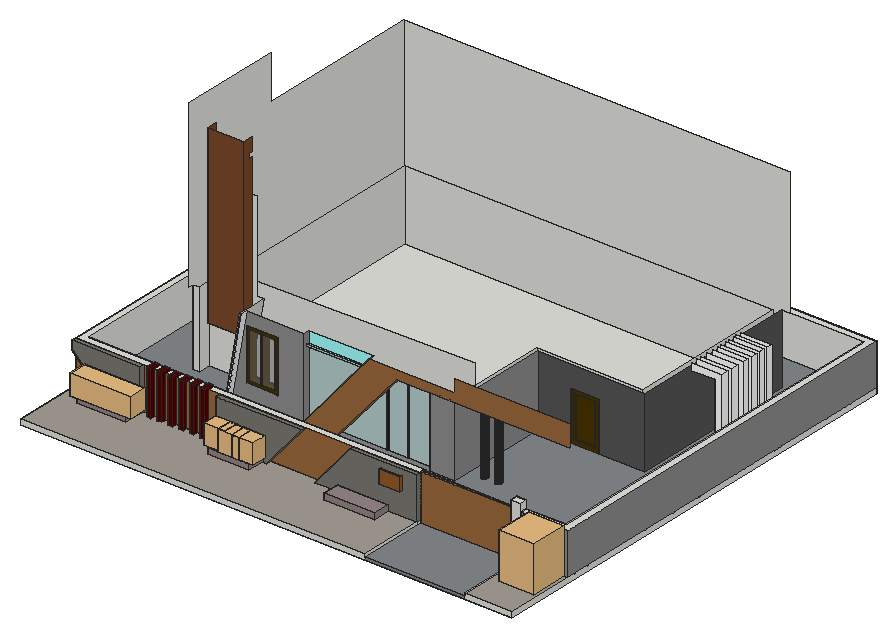
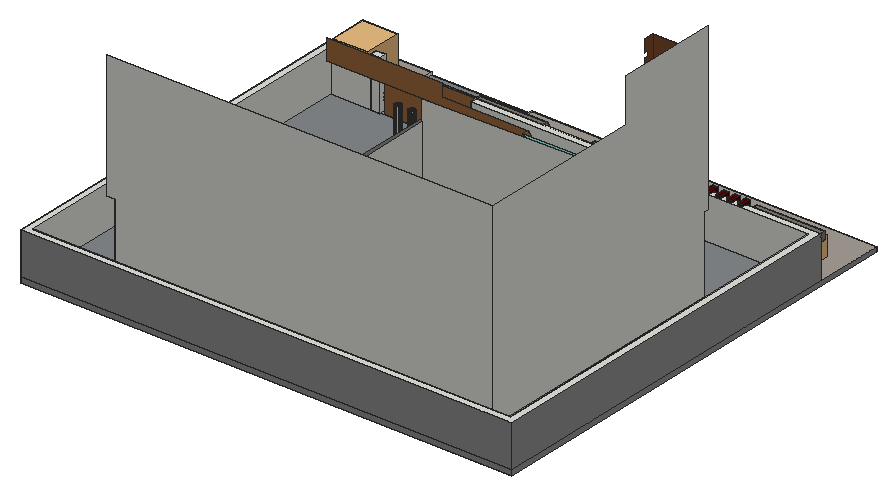
# SketchUp Ruby script. Lengths in inches.
U = 1.inch
M = Sketchup.active_model
def pt(a) = Geom::Point3d.new(a.map { |v| v * U })
def face(e, loops, mat)
  f = e.add_face(loops[0].map { |a| pt(a) })
  loops[1..].each { |l| e.add_face(l.map { |a| pt(a) }).erase! }
  f.material = f.back_material = mat if mat
  f
end
# faces: each face lists its corners as indices into pts; further lists are holes
def faces(e, pts, list, mat = nil) = list.each { |f| face(e, (f[0].is_a?(Array) ? f : [f]).map { |l| l.map { |i| pts[i] } }, mat) }
# xy, xz, yz: faces in a plane at the given z, y or x. An outline is a flat list of corners, or four numbers for a rectangle; further outlines are holes
def ring(l) = l.size == 4 ? [[l[0], l[1]], [l[2], l[1]], [l[2], l[3]], [l[0], l[3]]] : l.each_slice(2).to_a
def flat(e, list, mat, &to3) = list.each { |f| face(e, (f[0].is_a?(Array) ? f : [f]).map { |l| ring(l).map { |u, v| to3.(u, v) } }, mat) }
def xy(e, z, list, mat = nil) = flat(e, list, mat) { |x, y| [x, y, z] }
def xz(e, y, list, mat = nil) = flat(e, list, mat) { |x, z| [x, y, z] }
def yz(e, x, list, mat = nil) = flat(e, list, mat) { |y, z| [x, y, z] }
def lines(e, pts, list) = list.each { |a, b| e.add_line(pt(pts[a]), pt(pts[b])) }
# prism: a flat outline (further loops are holes) pulled along v
def prism(e, loops, v, mat = nil)
  f = face(e, loops, mat); d = Geom::Vector3d.new(v.map { |x| x * U })
  f.pushpull(f.normal.samedirection?(d) ? d.length : -d.length)
end
def box(e, o, s, mat = nil) = prism(e, [[o, [o[0] + s[0], o[1], o[2]], [o[0] + s[0], o[1] + s[1], o[2]], [o[0], o[1] + s[1], o[2]]]], [0, 0, s[2]], mat)
def at(x, y, z, deg = 0) = Geom::Transformation.translation(pt([x, y, z])) * Geom::Transformation.rotation(ORIGIN, Z_AXIS, deg.degrees)
def axes(o, x, y, z) = Geom::Transformation.new([*x, 0, *y, 0, *z, 0, *pt(o).to_a, 1])
def part(name) = M.definitions.add(name)
# library, detail: a bought-in or finely detailed component or shape, given as its bounding box
def library(name, o, s) = part(name).tap { |d| box(d.entities, o, s) }
def detail(e, o, s) = box(e.add_group.entities, o, s)
def put(e, d, t, mat = nil) = e.add_instance(d, t).tap { |i| i.material = mat if mat }
def group(e, t, mat = nil) = e.add_group.tap { |g| g.transformation = t; g.material = mat if mat }.entities
root = M.entities
M.materials.add("[Asphalt Stamped Brick]").color = [149, 133, 134]
M.materials.add("[Blacktop Old 01]").color = [132, 136, 139]
M.materials.add("[Carrera Marble]").color = [182, 207, 207]
M.materials.add("[Color A08]").color = [86, 0, 0]
M.materials.add("[Color C08]").color = [74, 51, 0]
M.materials.add("[Color H03]").color = [162, 255, 255]
M.materials.add("[Color M00]").color = [255, 255, 255]
M.materials.add("[Color M04]").color = [142, 142, 142]
M.materials.add("[Color M06]").color = [86, 86, 86]
M.materials.add("[Color M08]").color = [30, 30, 30]
M.materials.add("[Groundcover Sand Raked]").color = [165, 158, 150]
M.materials.add("[Rough Square Concrete Block]").color = [123, 120, 113]
M.materials.add("[Translucent Glass Gray]").color = [128, 128, 128]
M.materials["[Translucent Glass Gray]"].alpha = 0.5
M.materials.add("[Wood Floor Dark]").color = [123, 73, 42]
M.materials.add("[Wood Floor Parquet]").color = [145, 89, 39]
M.materials.add("[Wood Floor]").color = [155, 105, 61]
c1 = library("Plant\#1",[-5.68,0.72,0],[60.25,63.89,77.61])
c2 = library("FOLHAGEM DECORAÇÃO",[-6.77,-5.96,0],[13.85,12.76,12.48])
c3 = library("Group\#9",[0,0,0],[102.88,30.52,34.18])
xy(root,0,[[0,0,840,778.75]])
xy(root,4.5625,[[588.97,0,759.97,0,759.97,118.75,743.35,118.75,743.35,130.75,588.97,130.75]],"[Blacktop Old 01]")
xy(root,7.5625,[[126.8,110.75,134.92,116.58]],"[Color A08]")
xy(root,8.8125,[[163.67,110.75,171.8,116.58]],"[Color A08]")
xy(root,9,[[57.9,110.5625,115.8,118.75],[245.73,110.5625,333.45,118.75],[415,110.5625,564.34,118.75],[564.34,110.5625,588.97,118.75],[0,118.75,0,778.75,840,778.75,840,118.75,759.97,118.75,759.97,130.75,828,130.75,828,766.75,12,766.75,12,130.75,588.97,130.75,588.97,118.75],
  [743.35,118.75,759.97,130.75],[177.64,231,177.64,241.25,174.375,241.25,174.375,250.25,551.08,250.25,551.08,414.375,613.375,414.375,613.375,408.375,557.08,408.375,557.08,241.25,358.24,241.25,358.24,231],[514.48,231,557.08,241.25],[94.75,250.25,94.75,700.8125,741.0625,700.8125,741.0625,408.375,661.375,408.375,661.375,414.375,732.0625,414.375,732.0625,691.8125,103.75,691.8125,103.75,271.1875,105.9,271.1875,105.9,250.25],[174.375,250.25,551.08,250.25,551.08,281.3125,103.75,271.1875,174.375,271.1875],
  [582.5,258.46,581.04,258.72,579.69,259.34,578.55,260.29,577.7,261.51,577.18,262.9,577.05,264.38,577.3,265.84,577.93,267.1875,578.88,268.33,580.09,269.18,581.49,269.69,582.97,269.83,584.43,269.57,585.78,268.95,586.92,268,587.77,266.78,588.28,265.39,588.42,263.91,588.16,262.45,587.54,261.1,586.59,259.96,585.375,259.11,583.98,258.6],[605.875,258.46,604.41,258.72,603.07,259.34,601.93,260.29,601.07,261.51,600.56,262.9,600.43,264.38,600.68,265.84,601.3,267.1875,602.25,268.33,603.47,269.18,604.86,269.69,606.34,269.83,607.8,269.57,609.15,268.95,610.29,268,611.15,266.78,611.66,265.39,611.79,263.91,611.54,262.45,610.91,261.1,609.96,259.96,608.75,259.11,607.35,258.6],[103.75,271.1875,551.08,281.3125,551.08,414.375,732.0625,414.375,732.0625,691.8125,103.75,691.8125]])
xy(root,9,[[31.99,81.6875,115.8,110.5625],[255.9,81.6875,325.28,110.5625],[453.41,81.6875,540.22,110.5625]],"[Asphalt Stamped Brick]")
xy(root,9,[[[12,130.75,828,766.75],[174.375,220.625,174.375,271.1875,105.9,271.1875,105.9,250.25,94.75,250.25,94.75,700.8125,741.0625,700.8125,741.0625,408.375,661.375,408.375,661.375,414.375,613.375,414.375,613.375,408.375,557.08,408.375,557.08,231,514.48,231,514.48,241.25,471.69,241.25,471.69,240.4375,469.85,240.4375,469.85,241.25,436.25,241.25,436.25,240.4375,434.61,240.4375,434.61,241.25,358.24,241.25,358.24,231,177.64,231,177.64,220.625],[793.62,490.78,806.8125,502.66],[793.62,511.53,806.8125,523.41],[793.62,536.43,806.8125,546.3],[793.62,554.3,806.8125,564.18],[793.62,570.62,806.8125,580.49],[793.62,586.05,806.8125,595.93],[582.5,258.46,581.04,258.72,579.69,259.34,578.55,260.29,577.7,261.51,577.18,262.9,577.05,264.38,577.3,265.84,577.93,267.1875,578.88,268.33,580.09,269.18,581.49,269.69,582.97,269.83,584.43,269.57,585.78,268.95,586.92,268,587.77,266.78,588.28,265.39,588.42,263.91,588.16,262.45,587.54,261.1,586.59,259.96,585.375,259.11,583.98,258.6],[605.875,258.46,604.41,258.72,603.07,259.34,601.93,260.29,601.07,261.51,600.56,262.9,600.43,264.38,600.68,265.84,601.3,267.1875,602.25,268.33,603.47,269.18,604.86,269.69,606.34,269.83,607.8,269.57,609.15,268.95,610.29,268,611.15,266.78,611.66,265.39,611.79,263.91,611.54,262.45,610.91,261.1,609.96,259.96,608.75,259.11,607.35,258.6]]],"[Blacktop Old 01]")
xy(root,9,[[174.375,220.625,177.64,241.25]],"[Color M00]")
xy(root,9,[[434.61,240.4375,436.25,241.25],[469.85,240.4375,471.69,241.25]],"[Color M08]")
xy(root,9,[[[0,0,588.97,0,588.97,110.5625,540.22,110.5625,540.22,81.6875,453.41,81.6875,453.41,110.5625,415,110.5625,415,118.75,333.45,118.75,333.45,110.5625,325.28,110.5625,325.28,81.6875,255.9,81.6875,255.9,110.5625,245.73,110.5625,245.73,118.75,115.8,118.75,115.8,81.6875,31.99,81.6875,31.99,110.5625,57.9,110.5625,57.9,118.75,0,118.75],[145.23,110.75,153.36,116.58],[182.11,110.75,190.23,116.58],[200.55,110.75,208.67,116.58],[218.98,110.75,227.11,116.58]],[759.97,0,840,118.75]],"[Groundcover Sand Raked]")
xy(root,18.8125,[[31.99,81.6875,115.8,110.5625],[255.9,81.6875,325.28,110.5625],[453.41,81.6875,540.22,110.5625]],"[Asphalt Stamped Brick]")
xy(root,33.04,[[201.66,231,254.6,250.25]])
xy(root,48.51,[[527.14,106,563.34,110.5625]],"[Wood Floor Parquet]")
xy(root,70.88,[[527.14,106,563.34,110.5625]],"[Wood Floor Parquet]")
xy(root,81,[[0,118.75,126.8,118.75,126.8,127.97,134.92,127.97,134.92,118.75,145.23,118.75,145.23,127.97,153.36,127.97,153.36,118.75,163.67,118.75,163.67,127.97,171.8,127.97,171.8,118.75,182.11,118.75,182.11,127.97,190.23,127.97,190.23,118.75,200.55,118.75,200.55,127.97,208.67,127.97,208.67,118.75,218.98,118.75,218.98,127.97,227.11,127.97,227.11,118.75,588.97,118.75,588.97,130.75,12,130.75,12,766.75,828,766.75,828,130.75,759.97,130.75,759.97,118.75,840,118.75,840,778.75,0,778.75]])
xy(root,81,[[126.8,116.58,134.92,118.75],[145.23,116.58,153.36,118.75],[163.67,116.58,171.8,118.75],[182.11,116.58,190.23,118.75],[200.55,116.58,208.67,118.75],
  [218.98,116.58,227.11,118.75],[163.67,118.75,171.8,127.97],[182.11,118.75,190.23,127.97],[200.55,118.75,208.67,127.97],[218.98,118.75,227.11,127.97]],"[Color A08]")
xy(root,81,[[0,110.5625,115.8,118.75],[245.73,110.5625,393.07,118.75],[474.17,110.5625,588.97,118.75]],"[Rough Square Concrete Block]")
xy(root,84.3125,[[126.8,110.75,134.92,127.97],[145.23,110.75,153.36,127.97],[163.67,110.75,171.8,127.97],[182.11,110.75,190.23,127.97],[200.55,110.75,208.67,127.97],
  [218.98,110.75,227.11,127.97]],"[Color A08]")
xy(root,85.375,[[116.625,255.4375,178.1875,271.1875]])
xy(root,93,[[613.375,408.375,661.375,414.375]])
xy(root,94.25,[[743.35,118.75,759.97,130.75]])
xy(root,121.98,[[201.66,231,254.6,250.25]])
xy(root,122.22,[[299.43,236.6875,393.28,241.25]],"[Carrera Marble]")
xy(root,124.82,[[299.43,236.6875,395.4375,241.25]],"[Carrera Marble]")
xz(root,0,[[0,0,588.97,9],[759.97,0,840,9]])
xz(root,0,[[588.97,0,759.97,4.5625]],"[Blacktop Old 01]")
xz(root,81.6875,[[31.99,9,115.8,18.8125],[255.9,9,325.28,18.8125],[453.41,9,540.22,18.8125]],"[Asphalt Stamped Brick]")
xz(root,106,[[527.14,48.51,563.34,70.88]],"[Wood Floor Parquet]")
xz(root,110.5625,[[31.99,9,31.99,18.8125,48.09,18.8125,57.9,9],[57.9,9,115.8,18.8125],[255.9,9,325.28,18.8125],[453.41,9,540.22,18.8125]],"[Asphalt Stamped Brick]")
xz(root,110.5625,[[57.9,9,57.9,18.8125,48.09,18.8125],[245.73,9,255.9,9,255.9,18.8125,325.28,18.8125,325.28,9,333.45,9,393.07,81,245.73,81],[[415,9,453.41,9,453.41,18.8125,540.22,18.8125,540.22,9,588.97,9,588.97,81,474.17,81],[527.14,48.51,563.34,70.88]],[48.09,18.8125,115.8,18.8125,115.8,81,0,81,0,66.9]],"[Rough Square Concrete Block]")
xz(root,110.5625,[[527.14,48.51,563.34,70.88]],"[Wood Floor Parquet]")
xz(root,110.75,[[126.8,7.5625,134.92,84.3125],[163.67,8.8125,171.8,84.3125],[145.23,9,153.36,84.3125],[182.11,9,190.23,84.3125],[200.55,9,208.67,84.3125],
  [218.98,9,227.11,84.3125]],"[Color A08]")
xz(root,116.58,[[126.8,7.5625,134.92,81],[163.67,8.8125,171.8,81],[145.23,9,153.36,81],[182.11,9,190.23,81],[200.55,9,208.67,81],
  [218.98,9,227.11,81]],"[Color A08]")
xz(root,118.75,[[743.35,4.5625,759.97,9],[57.9,9,0,66.9,0,81,115.8,81,115.8,9],[245.73,9,245.73,81,393.07,81,333.45,9],[415,9,474.17,81,588.97,81,588.97,9],[743.35,9,759.97,94.25]])
xz(root,118.75,[[759.97,9,840,81]],"[Color M04]")
xz(root,118.75,[[0,9,57.9,9,0,66.9],[115.8,9,245.73,81],[333.45,9,415,9,474.17,81,393.07,81]],"[Wood Floor]")
xz(root,127.97,[[126.8,81,134.92,84.3125],[145.23,81,153.36,84.3125],[163.67,81,171.8,84.3125],[182.11,81,190.23,84.3125],[200.55,81,208.67,84.3125],
  [218.98,81,227.11,84.3125]],"[Color A08]")
xz(root,130.75,[[588.97,4.5625,743.35,9],[12,9,588.97,81],[743.35,9,759.97,94.25],[759.97,9,828,81]])
xz(root,220.625,[[174.375,9,177.64,9,201.89,143.5625,198.68,143.5625]],"[Color M00]")
xz(root,231,[[[177.64,9,201.89,143.5625,299.43,143.5625,299.43,9],[201.66,33.04,254.6,121.98]],[514.48,9,557.08,129]],"[Color M04]")
xz(root,231,[[299.43,9,358.24,9,458.61,129,754.5,129,754.5,165,557.08,165,557.08,143.5625,410.97,143.5625]],"[Wood Floor]")
xz(root,236.6875,[[299.43,122.22,393.28,122.22,395.4375,124.82,299.43,124.82]],"[Carrera Marble]")
xz(root,240.4375,[[434.61,9,436.25,9,436.25,102.26,434.61,100.3],[469.85,9,471.69,129]],"[Color M08]")
xz(root,241.25,[[299.43,9,393.28,122.22,299.43,122.22],[358.24,9,434.61,9,434.61,100.3],[436.25,9,469.85,9,469.85,129,458.61,129,436.25,102.26],[471.69,9,514.48,129]],"[Carrera Marble]")
xz(root,241.25,[[299.43,124.82,395.4375,124.82,410.97,143.5625,299.43,143.5625]],"[Color H03]")
xz(root,241.25,[[434.61,9,434.61,100.3,436.25,102.26,436.25,9],[469.85,9,471.69,129]],"[Color M08]")
xz(root,250.25,[[94.75,9,105.9,138.0625]])
xz(root,255.4375,[[116.625,85.375,178.1875,383.8125]],"[Wood Floor Dark]")
xz(root,271.1875,[[103.75,9,105.9,129],[105.9,9,174.375,9,198.68,143.5625,186.49,143.5625,186.49,297,178.1875,297,178.1875,85.375,116.625,85.375,116.625,357,105.9,357]])
xz(root,408.375,[[557.08,9,613.375,9,613.375,93,661.375,93,661.375,9,741.0625,9,741.0625,129,557.08,129]],"[Color M06]")
xz(root,414.375,[[551.08,9,551.08,129,732.0625,129,732.0625,9,661.375,9,661.375,93,613.375,93,613.375,9]])
xz(root,490.78,[[793.62,9,806.8125,9,806.8125,144.7,754.5,144.7,754.5,132.83,793.62,132.83]],"[Color M00]")
xz(root,502.66,[[793.62,9,793.62,132.83,754.5,132.83,754.5,144.7,806.8125,144.7,806.8125,9]],"[Color M00]")
xz(root,511.53,[[793.62,9,806.8125,9,806.8125,144.7,754.5,144.7,754.5,132.83,793.62,132.83]],"[Color M00]")
xz(root,523.41,[[793.62,9,793.62,132.83,754.5,132.83,754.5,144.7,806.8125,144.7,806.8125,9]],"[Color M00]")
xz(root,536.43,[[793.62,9,806.8125,9,806.8125,144.7,754.5625,144.7,754.5625,133.42,793.62,133.42]],"[Color M00]")
xz(root,546.3,[[793.62,9,793.62,133.42,754.5625,133.42,754.5625,144.7,806.8125,144.7,806.8125,9]],"[Color M00]")
xz(root,554.3,[[793.62,9,806.8125,9,806.8125,144.7,754.5625,144.7,754.5625,133.42,793.62,133.42]],"[Color M00]")
xz(root,564.18,[[793.62,9,793.62,133.42,754.5625,133.42,754.5625,144.7,806.8125,144.7,806.8125,9]],"[Color M00]")
xz(root,570.62,[[793.62,9,806.8125,9,806.8125,144.7,754.5625,144.7,754.5625,133.42,793.62,133.42]],"[Color M00]")
xz(root,580.49,[[793.62,9,793.62,133.42,754.5625,133.42,754.5625,144.7,806.8125,144.7,806.8125,9]],"[Color M00]")
xz(root,586.05,[[793.62,9,806.8125,9,806.8125,144.7,754.5625,144.7,754.5625,133.42,793.62,133.42]],"[Color M00]")
xz(root,595.93,[[793.62,9,793.62,133.42,754.5625,133.42,754.5625,144.7,806.8125,144.7,806.8125,9]],"[Color M00]")
xz(root,691.8125,[[103.75,9,732.0625,129]])
xz(root,700.8125,[[94.75,9,94.75,345,754.5,345,754.5,285,754.5625,285,754.5625,129,741.0625,129,741.0625,9]])
xz(root,766.75,[[12,9,828,81]])
xz(root,778.75,[[0,0,840,9],[0,9,840,81]],"[Color M04]")
yz(root,0,[[0,0,778.75,9],[118.75,9,778.75,81]],"[Color M04]")
yz(root,0,[[110.5625,66.9,118.75,81]],"[Rough Square Concrete Block]")
yz(root,12,[[130.75,9,766.75,81]])
yz(root,31.99,[[81.6875,9,110.5625,18.8125]],"[Asphalt Stamped Brick]")
yz(root,94.75,[[250.25,9,250.25,138.0625,241.25,138.0625,241.25,419.9375,415.6875,419.9375,415.6875,345,700.8125,345,700.8125,9]])
yz(root,103.75,[[271.1875,9,691.8125,129]])
yz(root,105.9,[[250.25,9,271.1875,138.0625]])
yz(root,115.8,[[81.6875,9,110.5625,18.8125]],"[Asphalt Stamped Brick]")
yz(root,115.8,[[110.5625,9,118.75,81]],"[Rough Square Concrete Block]")
yz(root,116.625,[[255.4375,85.375,271.1875,383.8125]],"[Wood Floor Dark]")
yz(root,126.8,[[110.75,7.5625,110.75,84.3125,127.97,84.3125,127.97,81,116.58,81,116.58,7.5625]],"[Color A08]")
yz(root,134.92,[[110.75,7.5625,116.58,7.5625,116.58,81,127.97,81,127.97,84.3125,110.75,84.3125]],"[Color A08]")
yz(root,145.23,[[110.75,9,110.75,84.3125,127.97,84.3125,127.97,81,116.58,81,116.58,9]],"[Color A08]")
yz(root,153.36,[[110.75,9,116.58,9,116.58,81,127.97,81,127.97,84.3125,110.75,84.3125]],"[Color A08]")
yz(root,163.67,[[110.75,8.8125,110.75,84.3125,127.97,84.3125,127.97,81,116.58,81,116.58,8.8125]],"[Color A08]")
yz(root,171.8,[[110.75,8.8125,116.58,8.8125,116.58,81,127.97,81,127.97,84.3125,110.75,84.3125]],"[Color A08]")
yz(root,178.1875,[[255.4375,85.375,271.1875,85.375,271.1875,354.375,264.5,354.375,264.5,362,271.1875,362,271.1875,383.8125,255.4375,383.8125]],"[Wood Floor Dark]")
yz(root,182.11,[[110.75,9,110.75,84.3125,127.97,84.3125,127.97,81,116.58,81,116.58,9]],"[Color A08]")
yz(root,190.23,[[110.75,9,116.58,9,116.58,81,127.97,81,127.97,84.3125,110.75,84.3125]],"[Color A08]")
yz(root,200.55,[[110.75,9,110.75,84.3125,127.97,84.3125,127.97,81,116.58,81,116.58,9]],"[Color A08]")
yz(root,201.66,[[231,33.04,250.25,121.98]])
yz(root,208.67,[[110.75,9,116.58,9,116.58,81,127.97,81,127.97,84.3125,110.75,84.3125]],"[Color A08]")
yz(root,218.98,[[110.75,9,110.75,84.3125,127.97,84.3125,127.97,81,116.58,81,116.58,9]],"[Color A08]")
yz(root,227.11,[[110.75,9,116.58,9,116.58,81,127.97,81,127.97,84.3125,110.75,84.3125]],"[Color A08]")
yz(root,245.73,[[110.5625,9,118.75,81]],"[Rough Square Concrete Block]")
yz(root,254.6,[[231,33.04,250.25,121.98]])
yz(root,255.9,[[81.6875,9,110.5625,18.8125]],"[Asphalt Stamped Brick]")
yz(root,299.43,[[231,9,231,143.5625,241.25,143.5625,241.25,124.82,236.6875,124.82,236.6875,122.22,241.25,122.22,241.25,9]],"[Color M04]")
yz(root,325.28,[[81.6875,9,110.5625,18.8125]],"[Asphalt Stamped Brick]")
yz(root,434.61,[[240.4375,9,241.25,100.3]],"[Color M08]")
yz(root,436.25,[[240.4375,9,241.25,102.26]],"[Color M08]")
yz(root,453.41,[[81.6875,9,110.5625,18.8125]],"[Asphalt Stamped Brick]")
yz(root,469.85,[[240.4375,9,241.25,129]],"[Color M08]")
yz(root,471.69,[[240.4375,9,241.25,129]],"[Color M08]")
yz(root,514.48,[[231,9,241.25,129]],"[Color M04]")
yz(root,527.14,[[106,48.51,110.5625,70.88]],"[Wood Floor Parquet]")
yz(root,540.22,[[81.6875,9,110.5625,18.8125]],"[Asphalt Stamped Brick]")
yz(root,551.08,[[250.25,9,281.3125,129],[281.3125,9,414.375,129]])
yz(root,557.08,[[231,9,408.375,129]],"[Color M04]")
yz(root,563.34,[[106,48.51,110.5625,70.88]],"[Wood Floor Parquet]")
yz(root,588.97,[[0,4.5625,110.5625,9],[110.5625,4.5625,118.75,9],[118.75,4.5625,130.75,9],[118.75,9,130.75,81]])
yz(root,588.97,[[110.5625,9,118.75,81]],"[Rough Square Concrete Block]")
yz(root,613.375,[[408.375,9,414.375,93]])
yz(root,661.375,[[408.375,9,414.375,93]])
yz(root,732.0625,[[414.375,9,691.8125,129]])
yz(root,741.0625,[[408.375,9,700.8125,129]],"[Color M06]")
yz(root,743.35,[[118.75,4.5625,130.75,9],[118.75,9,130.75,94.25]])
yz(root,759.97,[[0,4.5625,118.75,9],[118.75,9,130.75,81],[118.75,81,130.75,94.25]])
yz(root,793.62,[[490.78,9,502.66,132.83],[511.53,9,523.41,132.83],[536.43,9,546.3,133.42],[554.3,9,564.18,133.42],[570.62,9,580.49,133.42],
  [586.05,9,595.93,133.42]],"[Color M00]")
yz(root,806.8125,[[490.78,9,502.66,144.7],[511.53,9,523.41,144.7],[536.43,9,546.3,144.7],[554.3,9,564.18,144.7],[570.62,9,580.49,144.7],
  [586.05,9,595.93,144.7]],"[Color M00]")
yz(root,828,[[130.75,9,766.75,81]])
yz(root,840,[[0,0,778.75,9]])
yz(root,840,[[118.75,9,778.75,81]],"[Color M04]")
p = [[0,118.75,66.9],[57.9,118.75,9],[57.9,110.5625,9],[48.09,110.5625,18.8125],[0,110.5625,66.9],[333.45,118.75,9],
  [393.07,118.75,81],[393.07,110.5625,81],[333.45,110.5625,9],[474.17,118.75,81],[415,118.75,9],[415,110.5625,9],
  [474.17,110.5625,81],[198.68,220.625,143.5625],[198.68,241.25,143.5625],[198.68,271.1875,143.5625],[174.375,271.1875,9],[174.375,250.25,9],
  [174.375,241.25,9],[174.375,220.625,9],[177.64,220.625,9],[177.64,231,9],[201.89,231,143.5625],[201.89,220.625,143.5625],
  [393.28,241.25,122.22],[299.43,241.25,9],[299.43,231,9],[410.97,231,143.5625],[410.97,241.25,143.5625],[395.4375,241.25,124.82],
  [395.4375,236.6875,124.82],[393.28,236.6875,122.22],[358.24,241.25,9],[434.61,241.25,100.3],[434.61,240.4375,100.3],[436.25,240.4375,102.26],
  [436.25,241.25,102.26],[458.61,241.25,129],[458.61,231,129],[358.24,231,9],[581.04,258.72,9],[582.5,258.46,9],
  [582.5,258.46,129],[581.04,258.72,129],[583.98,258.6,9],[583.98,258.6,129],[604.41,258.72,9],[605.875,258.46,9],
  [605.875,258.46,129],[604.41,258.72,129],[607.35,258.6,9],[607.35,258.6,129],[585.375,259.11,9],[585.375,259.11,129],
  [608.75,259.11,9],[608.75,259.11,129],[579.69,259.34,9],[579.69,259.34,129],[603.07,259.34,9],[603.07,259.34,129],
  [586.59,259.96,9],[586.59,259.96,129],[609.96,259.96,9],[609.96,259.96,129],[578.55,260.29,9],[578.55,260.29,129],
  [601.93,260.29,9],[601.93,260.29,129],[587.54,261.1,9],[587.54,261.1,129],[610.91,261.1,9],[610.91,261.1,129],
  [577.7,261.51,9],[577.7,261.51,129],[601.07,261.51,9],[601.07,261.51,129],[588.16,262.45,9],[588.16,262.45,129],
  [611.54,262.45,9],[611.54,262.45,129],[577.18,262.9,9],[577.18,262.9,129],[600.56,262.9,9],[600.56,262.9,129],
  [588.42,263.91,9],[588.42,263.91,129],[611.79,263.91,9],[611.79,263.91,129],[577.05,264.38,9],[577.05,264.38,129],
  [600.43,264.38,9],[600.43,264.38,129],[588.28,265.39,9],[588.28,265.39,129],[611.66,265.39,9],[611.66,265.39,129],
  [577.3,265.84,9],[577.3,265.84,129],[600.68,265.84,9],[600.68,265.84,129],[587.77,266.78,9],[587.77,266.78,129],
  [611.15,266.78,9],[611.15,266.78,129],[577.93,267.1875,9],[577.93,267.1875,129],[601.3,267.1875,9],[601.3,267.1875,129],
  [586.92,268,9],[586.92,268,129],[610.29,268,9],[610.29,268,129],[578.88,268.33,9],[578.88,268.33,129],
  [602.25,268.33,9],[602.25,268.33,129],[585.78,268.95,9],[585.78,268.95,129],[609.15,268.95,9],[609.15,268.95,129],
  [580.09,269.18,9],[580.09,269.18,129],[603.47,269.18,9],[603.47,269.18,129],[584.43,269.57,9],[584.43,269.57,129],
  [607.8,269.57,9],[607.8,269.57,129],[581.49,269.69,9],[581.49,269.69,129],[604.86,269.69,9],[604.86,269.69,129],
  [582.97,269.83,9],[582.97,269.83,129],[606.34,269.83,9],[606.34,269.83,129],[103.75,271.1875,165],[551.08,281.3125,165],
  [551.08,281.3125,133],[551.08,281.3125,129],[551.08,281.3125,9],[103.75,271.1875,9],[103.75,271.1875,129],[103.75,271.1875,133]]
faces(root,p,[[0,1,2,3,4],[5,6,7,8],[9,10,11,12]],"[Rough Square Concrete Block]")
faces(root,p,[[13,14,15,16,17,18,19],[40,41,42,43],[41,44,45,42],[46,47,48,49],[47,50,51,48],[44,52,53,45],[50,54,55,51],[56,40,43,57],
  [58,46,49,59],[52,60,61,53],[54,62,63,55],[64,56,57,65],[66,58,59,67],[60,68,69,61],[62,70,71,63],[72,64,65,73],
  [74,66,67,75],[68,76,77,69],[70,78,79,71],[80,72,73,81],[82,74,75,83],[76,84,85,77],[78,86,87,79],[88,80,81,89],
  [90,82,83,91],[84,92,93,85],[86,94,95,87],[96,88,89,97],[98,90,91,99],[92,100,101,93],[94,102,103,95],[104,96,97,105],
  [106,98,99,107],[100,108,109,101],[102,110,111,103],[112,104,105,113],[114,106,107,115],[108,116,117,109],[110,118,119,111],[120,112,113,121],
  [122,114,115,123],[116,124,125,117],[118,126,127,119],[128,120,121,129],[130,122,123,131],[124,132,133,125],[126,134,135,127],[132,128,129,133],
  [134,130,131,135],[136,137,138,139,140,141,142,143]])
faces(root,p,[[20,21,22,23]],"[Color M00]")
faces(root,p,[[24,25,26,27,28,29,30,31],[32,33,34,35,36,37,38,39]],"[Wood Floor]")
faces(root,p,[[33,36,35,34]],"[Color M08]")
g1 = group(root,at(588.97,118.75,4.5625))
box(g1,[0,0,0],[154.38,4,78.71],"[Wood Floor]")
put(root,c1,at(779.6,54.14,9))
g2 = group(root,at(613.375,408.375,9))
xy(g2,0,[[0,0,48,9.5625]],"[Color C08]")
xy(g2,6.07,[[6.07,0,41.93,3.5625],[6.07,3.5625,41.93,9.5625]],"[Color C08]")
xy(g2,77.93,[[6.07,0,41.93,3.5625],[6.07,3.5625,41.93,9.5625]],"[Color C08]")
xy(g2,84,[[0,0,48,9.5625]],"[Color C08]")
xz(g2,0,[[[0,0,48,84],[6.07,6.07,41.93,77.93]]],"[Color C08]")
xz(g2,3.5625,[[6.07,6.07,41.93,77.93]],"[Color C08]")
xz(g2,9.5625,[[[0,0,48,84],[6.07,6.07,41.93,77.93]],[6.07,6.07,41.93,77.93]],"[Color C08]")
yz(g2,0,[[0,0,9.5625,84]],"[Color C08]")
yz(g2,6.07,[[0,6.07,3.5625,77.93],[3.5625,6.07,9.5625,77.93]],"[Color C08]")
yz(g2,41.93,[[0,6.07,3.5625,77.93],[3.5625,6.07,9.5625,77.93]],"[Color C08]")
yz(g2,48,[[0,0,9.5625,84]],"[Color C08]")
put(root,c2,axes([263.99,95.71,18.8125],[2.59,0,0],[0,2,0],[0,0,2.74]))
put(root,c2,axes([289.55,93.6,18.8125],[2.59,0,0],[0,2,0],[0,0,2.74]))
put(root,c2,axes([313.05,93.6,18.8125],[2.59,0,0],[0,2,0],[0,0,2.74]))
put(root,c3,at(22.98,77.95,18.8125))
g3 = group(root,at(201.66,231,33.04))
xy(g3,0,[[0,0,52.9375,13.4]],"[Color C08]")
xy(g3,5.23,[[5.04,0,25.13,13.4],[25.13,0,27.58,13.4],[27.58,0,47.9,13.4]],"[Color C08]")
xy(g3,83.71,[[5.04,0,25.13,13.4],[25.13,0,27.58,13.4],[27.58,0,47.9,13.4]],"[Color C08]")
xy(g3,88.9375,[[0,0,52.9375,13.4]],"[Color C08]")
xz(g3,0,[[[0,0,52.9375,88.9375],[5.04,5.23,47.9,83.71]],[25.13,5.23,27.58,83.71]],"[Color C08]")
xz(g3,0,[[5.04,5.23,25.13,83.71],[27.58,5.23,47.9,83.71]],"[Translucent Glass Gray]")
xz(g3,13.4,[[[0,0,52.9375,88.9375],[5.04,5.23,47.9,83.71]],[25.13,5.23,27.58,83.71]],"[Color C08]")
yz(g3,0,[[0,0,13.4,88.9375]],"[Color C08]")
yz(g3,5.04,[[0,5.23,13.4,83.71]],"[Color C08]")
yz(g3,25.13,[[0,5.23,13.4,83.71]],"[Color C08]")
yz(g3,27.58,[[0,5.23,13.4,83.71]],"[Color C08]")
yz(g3,47.9,[[0,5.23,13.4,83.71]],"[Color C08]")
yz(g3,52.9375,[[0,0,13.4,88.9375]],"[Color C08]")
